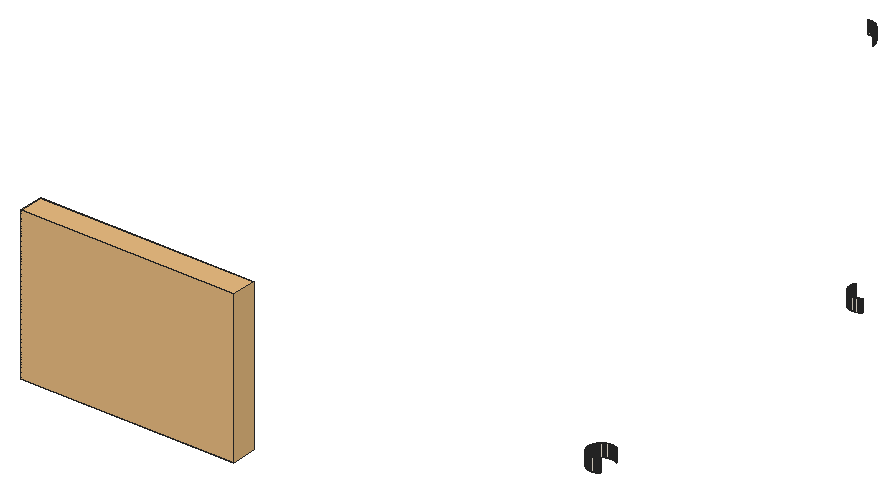
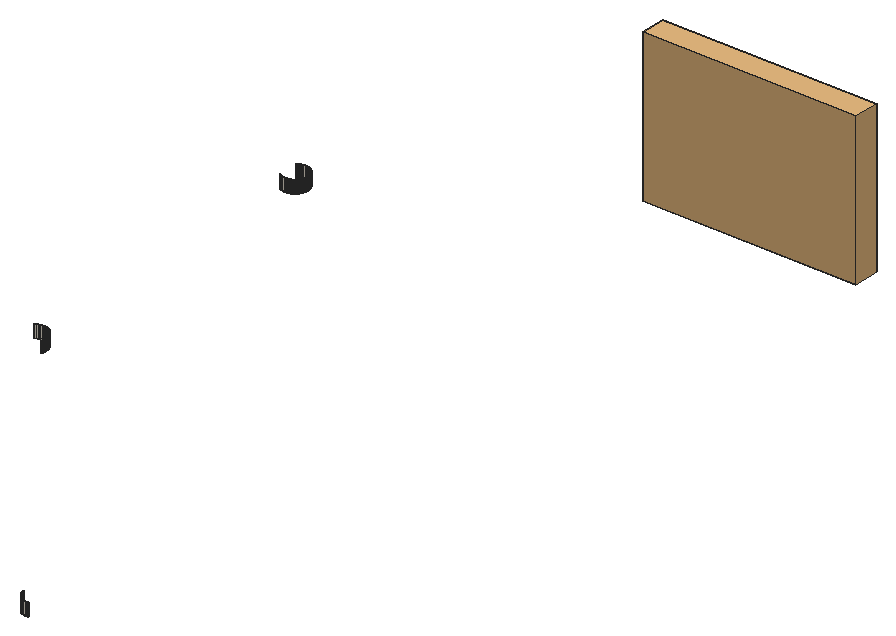
# SketchUp Ruby script. Lengths in inches.
U = 1.inch
M = Sketchup.active_model
def pt(a) = Geom::Point3d.new(a.map { |v| v * U })
def face(e, loops, mat)
  f = e.add_face(loops[0].map { |a| pt(a) })
  loops[1..].each { |l| e.add_face(l.map { |a| pt(a) }).erase! }
  f.material = f.back_material = mat if mat
  f
end
# faces: each face lists its corners as indices into pts; further lists are holes
def faces(e, pts, list, mat = nil) = list.each { |f| face(e, (f[0].is_a?(Array) ? f : [f]).map { |l| l.map { |i| pts[i] } }, mat) }
# xy, xz, yz: faces in a plane at the given z, y or x. An outline is a flat list of corners, or four numbers for a rectangle; further outlines are holes
def ring(l) = l.size == 4 ? [[l[0], l[1]], [l[2], l[1]], [l[2], l[3]], [l[0], l[3]]] : l.each_slice(2).to_a
def flat(e, list, mat, &to3) = list.each { |f| face(e, (f[0].is_a?(Array) ? f : [f]).map { |l| ring(l).map { |u, v| to3.(u, v) } }, mat) }
def xy(e, z, list, mat = nil) = flat(e, list, mat) { |x, y| [x, y, z] }
def xz(e, y, list, mat = nil) = flat(e, list, mat) { |x, z| [x, y, z] }
def yz(e, x, list, mat = nil) = flat(e, list, mat) { |y, z| [x, y, z] }
def lines(e, pts, list) = list.each { |a, b| e.add_line(pt(pts[a]), pt(pts[b])) }
# prism: a flat outline (further loops are holes) pulled along v
def prism(e, loops, v, mat = nil)
  f = face(e, loops, mat); d = Geom::Vector3d.new(v.map { |x| x * U })
  f.pushpull(f.normal.samedirection?(d) ? d.length : -d.length)
end
def box(e, o, s, mat = nil) = prism(e, [[o, [o[0] + s[0], o[1], o[2]], [o[0] + s[0], o[1] + s[1], o[2]], [o[0], o[1] + s[1], o[2]]]], [0, 0, s[2]], mat)
def at(x, y, z, deg = 0) = Geom::Transformation.translation(pt([x, y, z])) * Geom::Transformation.rotation(ORIGIN, Z_AXIS, deg.degrees)
def axes(o, x, y, z) = Geom::Transformation.new([*x, 0, *y, 0, *z, 0, *pt(o).to_a, 1])
def part(name) = M.definitions.add(name)
# library, detail: a bought-in or finely detailed component or shape, given as its bounding box
def library(name, o, s) = part(name).tap { |d| box(d.entities, o, s) }
def detail(e, o, s) = box(e.add_group.entities, o, s)
def put(e, d, t, mat = nil) = e.add_instance(d, t).tap { |i| i.material = mat if mat }
def group(e, t, mat = nil) = e.add_group.tap { |g| g.transformation = t; g.material = mat if mat }.entities
root = M.entities
M.materials.add("0027 AP L140 CRUSHED ICE").color = [241, 233, 217]
c1 = library("Group\#28",[0,0,-12],[51,6,35.99])
xz(root,255,[[122.84,120,122.92,123],[122.92,120,123,123],[123,120,123.08,123],[123.08,120,123.16,123]],"0027 AP L140 CRUSHED ICE")
xz(root,261,[[122.84,120,122.92,123],[122.92,120,123,123],[123,120,123.08,123],[123.08,120,123.16,123]],"0027 AP L140 CRUSHED ICE")
xz(root,333,[[122.84,120,122.92,123],[122.92,120,123,123],[123,120,123.08,123],[123.08,120,123.16,123]],"0027 AP L140 CRUSHED ICE")
xz(root,417,[[59.84,120,59.92,123],[59.92,120,60,123],[60,120,60.08,123],[60.08,120,60.16,123]],"0027 AP L140 CRUSHED ICE")
yz(root,63,[[414,120,414.08,123],[414.08,120,414.16,123]],"0027 AP L140 CRUSHED ICE")
yz(root,120,[[257.84,120,257.92,123],[257.92,120,258,123],[258,120,258.08,123],[258.08,120,258.16,123],[335.84,120,335.92,123],
  [335.92,120,336,123],[336,120,336.08,123],[336.08,120,336.16,123]],"0027 AP L140 CRUSHED ICE")
p = [[122.53,255.04,120],[122.45,255.05,120],[122.45,255.05,123],[122.53,255.04,123],[122.61,255.03,120],[122.61,255.03,123],
  [122.6875,255.02,120],[122.6875,255.02,123],[122.76,255.01,120],[122.76,255.01,123],[122.84,255,120],[122.84,255,123],
  [123.24,255.01,120],[123.16,255,120],[123.16,255,123],[123.24,255.01,123],[123.3125,255.02,120],[123.3125,255.02,123],
  [123.39,255.03,120],[123.39,255.03,123],[123.47,255.04,120],[123.47,255.04,123],[123.55,255.05,120],[123.55,255.05,123],
  [122.07,255.15,120],[122,255.17,120],[122,255.17,123],[122.07,255.15,123],[122.15,255.125,120],[122.15,255.125,123],
  [122.22,255.1,120],[122.22,255.1,123],[122.3,255.08,120],[122.3,255.08,123],[122.375,255.07,120],[122.375,255.07,123],
  [123.625,255.07,120],[123.625,255.07,123],[123.7,255.08,120],[123.7,255.08,123],[123.78,255.1,120],[123.78,255.1,123],
  [123.85,255.125,120],[123.85,255.125,123],[123.93,255.15,120],[123.93,255.15,123],[124,255.17,120],[124,255.17,123],
  [121.85,255.23,120],[121.78,255.26,120],[121.78,255.26,123],[121.85,255.23,123],[121.92,255.2,120],[121.92,255.2,123],
  [124.08,255.2,120],[124.08,255.2,123],[124.15,255.23,120],[124.15,255.23,123],[124.22,255.26,120],[124.22,255.26,123],
  [121.64,255.33,120],[121.57,255.36,120],[121.57,255.36,123],[121.64,255.33,123],[121.71,255.29,120],[121.71,255.29,123],
  [124.29,255.29,120],[124.29,255.29,123],[124.36,255.33,120],[124.36,255.33,123],[124.43,255.36,120],[124.43,255.36,123],
  [121.43,255.44,120],[121.37,255.48,120],[121.37,255.48,123],[121.43,255.44,123],[121.5,255.4,120],[121.5,255.4,123],
  [124.5,255.4,120],[124.5,255.4,123],[124.57,255.44,120],[124.57,255.44,123],[124.63,255.48,120],[124.63,255.48,123],
  [121.3,255.53,120],[121.24,255.57,120],[121.24,255.57,123],[121.3,255.53,123],[124.7,255.53,120],[124.7,255.53,123],
  [124.76,255.57,120],[124.76,255.57,123],[121.17,255.62,120],[121.11,255.67,120],[121.11,255.67,123],[121.17,255.62,123],
  [124.83,255.62,120],[124.83,255.62,123],[124.89,255.67,120],[124.89,255.67,123],[121.05,255.72,120],[120.99,255.77,120],
  [120.99,255.77,123],[121.05,255.72,123],[120.93,255.82,120],[120.88,255.88,120],[120.88,255.88,123],[120.93,255.82,123],
  [120.82,255.93,120],[120.77,255.99,120],[120.77,255.99,123],[120.82,255.93,123],[120.72,256.05,120],[120.72,256.05,123],
  [120.67,256.11,120],[120.62,256.17,120],[120.62,256.17,123],[120.67,256.11,123],[120.57,256.24,120],[120.53,256.3,120],
  [120.53,256.3,123],[120.57,256.24,123],[120.48,256.37,120],[120.48,256.37,123],[120.44,256.43,120],[120.4,256.5,120],
  [120.4,256.5,123],[120.44,256.43,123],[120.36,256.57,120],[120.36,256.57,123],[120.33,256.64,120],[120.29,256.71,120],
  [120.29,256.71,123],[120.33,256.64,123],[120.26,256.78,120],[120.26,256.78,123],[120.23,256.85,120],[120.23,256.85,123],
  [120.2,256.92,120],[120.17,257,120],[120.17,257,123],[120.2,256.92,123],[120.15,257.07,120],[120.15,257.07,123],
  [120.125,257.15,120],[120.1,257.22,120],[120.1,257.22,123],[120.125,257.15,123],[120.08,257.3,120],[120.08,257.3,123],
  [120.07,257.375,120],[120.07,257.375,123],[120.05,257.45,120],[120.05,257.45,123],[120.04,257.53,120],[120.03,257.61,120],
  [120.03,257.61,123],[120.04,257.53,123],[120.02,257.6875,120],[120.02,257.6875,123],[120.01,257.76,120],[120.01,257.76,123],
  [120,257.84,120],[120,257.84,123],[120,258.16,120],[120.01,258.24,120],[120.01,258.24,123],[120,258.16,123],
  [120.02,258.3125,120],[120.02,258.3125,123],[120.03,258.39,120],[120.03,258.39,123],[120.04,258.47,120],[120.04,258.47,123],
  [120.05,258.55,120],[120.05,258.55,123],[120.07,258.625,120],[120.07,258.625,123],[120.08,258.7,120],[120.08,258.7,123],
  [120.1,258.78,120],[120.1,258.78,123],[120.125,258.85,120],[120.125,258.85,123],[120.15,258.93,120],[120.15,258.93,123],
  [120.17,259,120],[120.17,259,123],[120.2,259.08,120],[120.2,259.08,123],[120.23,259.15,120],[120.23,259.15,123],
  [120.26,259.22,120],[120.26,259.22,123],[120.29,259.29,120],[120.29,259.29,123],[120.33,259.36,120],[120.33,259.36,123],
  [120.36,259.43,120],[120.36,259.43,123],[120.4,259.5,120],[120.4,259.5,123],[120.44,259.57,120],[120.44,259.57,123],
  [120.48,259.63,120],[120.48,259.63,123],[120.53,259.7,120],[120.53,259.7,123],[120.57,259.76,120],[120.57,259.76,123],
  [120.62,259.83,120],[120.62,259.83,123],[120.67,259.89,120],[120.67,259.89,123],[120.72,259.95,120],[120.72,259.95,123],
  [120.77,260.01,120],[120.77,260.01,123],[120.82,260.07,120],[120.82,260.07,123],[120.88,260.12,120],[120.88,260.12,123],
  [120.93,260.18,120],[120.93,260.18,123],[120.99,260.23,120],[120.99,260.23,123],[121.05,260.28,120],[121.05,260.28,123],
  [121.11,260.33,120],[121.11,260.33,123],[121.17,260.38,120],[121.17,260.38,123],[124.83,260.38,120],[124.89,260.33,120],
  [124.89,260.33,123],[124.83,260.38,123],[121.24,260.43,120],[121.24,260.43,123],[121.3,260.47,120],[121.3,260.47,123],
  [124.7,260.47,120],[124.76,260.43,120],[124.76,260.43,123],[124.7,260.47,123],[121.37,260.52,120],[121.37,260.52,123],
  [121.43,260.56,120],[121.43,260.56,123],[124.57,260.56,120],[124.63,260.52,120],[124.63,260.52,123],[124.57,260.56,123],
  [121.5,260.6,120],[121.5,260.6,123],[121.57,260.64,120],[121.57,260.64,123],[121.64,260.67,120],[121.64,260.67,123],
  [124.36,260.67,120],[124.43,260.64,120],[124.43,260.64,123],[124.36,260.67,123],[124.5,260.6,120],[124.5,260.6,123],
  [121.71,260.71,120],[121.71,260.71,123],[121.78,260.74,120],[121.78,260.74,123],[121.85,260.77,120],[121.85,260.77,123],
  [124.15,260.77,120],[124.22,260.74,120],[124.22,260.74,123],[124.15,260.77,123],[124.29,260.71,120],[124.29,260.71,123],
  [121.92,260.8,120],[121.92,260.8,123],[122,260.83,120],[122,260.83,123],[122.07,260.85,120],[122.07,260.85,123],
  [123.93,260.85,120],[124,260.83,120],[124,260.83,123],[123.93,260.85,123],[124.08,260.8,120],[124.08,260.8,123],
  [122.15,260.875,120],[122.15,260.875,123],[122.22,260.9,120],[122.22,260.9,123],[122.3,260.92,120],[122.3,260.92,123],
  [122.375,260.93,120],[122.375,260.93,123],[122.45,260.95,120],[122.45,260.95,123],[122.53,260.96,120],[122.53,260.96,123],
  [123.47,260.96,120],[123.55,260.95,120],[123.55,260.95,123],[123.47,260.96,123],[123.625,260.93,120],[123.625,260.93,123],
  [123.7,260.92,120],[123.7,260.92,123],[123.78,260.9,120],[123.78,260.9,123],[123.85,260.875,120],[123.85,260.875,123],
  [122.61,260.97,120],[122.61,260.97,123],[122.6875,260.98,120],[122.6875,260.98,123],[122.76,260.99,120],[122.76,260.99,123],
  [122.84,261,120],[122.84,261,123],[123.16,261,120],[123.24,260.99,120],[123.24,260.99,123],[123.16,261,123],
  [123.3125,260.98,120],[123.3125,260.98,123],[123.39,260.97,120],[123.39,260.97,123],[122.53,333.04,120],[122.45,333.05,120],
  [122.45,333.05,123],[122.53,333.04,123],[122.61,333.03,120],[122.61,333.03,123],[122.6875,333.02,120],[122.6875,333.02,123],
  [122.76,333.01,120],[122.76,333.01,123],[122.84,333,120],[122.84,333,123],[123.24,333.01,120],[123.16,333,120],
  [123.16,333,123],[123.24,333.01,123],[123.3125,333.02,120],[123.3125,333.02,123],[123.39,333.03,120],[123.39,333.03,123],
  [123.47,333.04,120],[123.47,333.04,123],[123.55,333.05,120],[123.55,333.05,123],[122.07,333.15,120],[122,333.17,120],
  [122,333.17,123],[122.07,333.15,123],[122.15,333.125,120],[122.15,333.125,123],[122.22,333.1,120],[122.22,333.1,123],
  [122.3,333.08,120],[122.3,333.08,123],[122.375,333.07,120],[122.375,333.07,123],[123.625,333.07,120],[123.625,333.07,123],
  [123.7,333.08,120],[123.7,333.08,123],[123.78,333.1,120],[123.78,333.1,123],[123.85,333.125,120],[123.85,333.125,123],
  [123.93,333.15,120],[123.93,333.15,123],[124,333.17,120],[124,333.17,123],[121.85,333.23,120],[121.78,333.26,120],
  [121.78,333.26,123],[121.85,333.23,123],[121.92,333.2,120],[121.92,333.2,123],[124.08,333.2,120],[124.08,333.2,123],
  [124.15,333.23,120],[124.15,333.23,123],[124.22,333.26,120],[124.22,333.26,123],[121.64,333.33,120],[121.57,333.36,120],
  [121.57,333.36,123],[121.64,333.33,123],[121.71,333.29,120],[121.71,333.29,123],[124.29,333.29,120],[124.29,333.29,123],
  [124.36,333.33,120],[124.36,333.33,123],[124.43,333.36,120],[124.43,333.36,123],[121.43,333.44,120],[121.37,333.48,120],
  [121.37,333.48,123],[121.43,333.44,123],[121.5,333.4,120],[121.5,333.4,123],[124.5,333.4,120],[124.5,333.4,123],
  [124.57,333.44,120],[124.57,333.44,123],[124.63,333.48,120],[124.63,333.48,123],[121.3,333.53,120],[121.24,333.57,120],
  [121.24,333.57,123],[121.3,333.53,123],[124.7,333.53,120],[124.7,333.53,123],[124.76,333.57,120],[124.76,333.57,123],
  [121.17,333.62,120],[121.11,333.67,120],[121.11,333.67,123],[121.17,333.62,123],[124.83,333.62,120],[124.83,333.62,123],
  [124.89,333.67,120],[124.89,333.67,123],[121.05,333.72,120],[120.99,333.77,120],[120.99,333.77,123],[121.05,333.72,123],
  [120.93,333.82,120],[120.88,333.88,120],[120.88,333.88,123],[120.93,333.82,123],[120.82,333.93,120],[120.77,333.99,120],
  [120.77,333.99,123],[120.82,333.93,123],[120.72,334.05,120],[120.72,334.05,123],[120.67,334.11,120],[120.62,334.17,120],
  [120.62,334.17,123],[120.67,334.11,123],[120.57,334.24,120],[120.53,334.3,120],[120.53,334.3,123],[120.57,334.24,123],
  [120.48,334.37,120],[120.48,334.37,123],[120.44,334.43,120],[120.4,334.5,120],[120.4,334.5,123],[120.44,334.43,123],
  [120.36,334.57,120],[120.36,334.57,123],[120.33,334.64,120],[120.29,334.71,120],[120.29,334.71,123],[120.33,334.64,123],
  [120.26,334.78,120],[120.26,334.78,123],[120.23,334.85,120],[120.23,334.85,123],[120.2,334.92,120],[120.17,335,120],
  [120.17,335,123],[120.2,334.92,123],[120.15,335.07,120],[120.15,335.07,123],[120.125,335.15,120],[120.1,335.22,120],
  [120.1,335.22,123],[120.125,335.15,123],[120.08,335.3,120],[120.08,335.3,123],[120.07,335.375,120],[120.07,335.375,123],
  [120.05,335.45,120],[120.05,335.45,123],[120.04,335.53,120],[120.03,335.61,120],[120.03,335.61,123],[120.04,335.53,123],
  [120.02,335.6875,120],[120.02,335.6875,123],[120.01,335.76,120],[120.01,335.76,123],[120,335.84,120],[120,335.84,123],
  [120,336.16,120],[120.01,336.24,120],[120.01,336.24,123],[120,336.16,123],[120.02,336.3125,120],[120.02,336.3125,123],
  [120.03,336.39,120],[120.03,336.39,123],[120.04,336.47,120],[120.04,336.47,123],[120.05,336.55,120],[120.05,336.55,123],
  [120.07,336.625,120],[120.07,336.625,123],[120.08,336.7,120],[120.08,336.7,123],[120.1,336.78,120],[120.1,336.78,123],
  [120.125,336.85,120],[120.125,336.85,123],[120.15,336.93,120],[120.15,336.93,123],[120.17,337,120],[120.17,337,123],
  [120.2,337.08,120],[120.2,337.08,123],[120.23,337.15,120],[120.23,337.15,123],[120.26,337.22,120],[120.26,337.22,123],
  [62.98,414.3125,120],[62.99,414.24,120],[62.99,414.24,123],[62.98,414.3125,123],[63,414.16,120],[63,414.16,123],
  [62.97,414.39,120],[62.97,414.39,123],[62.96,414.47,120],[62.96,414.47,123],[62.93,414.625,120],[62.95,414.55,120],
  [62.95,414.55,123],[62.93,414.625,123],[62.92,414.7,120],[62.92,414.7,123],[62.9,414.78,120],[62.9,414.78,123],
  [62.875,414.85,120],[62.875,414.85,123],[62.83,415,120],[62.85,414.93,120],[62.85,414.93,123],[62.83,415,123],
  [62.8,415.08,120],[62.8,415.08,123],[62.74,415.22,120],[62.77,415.15,120],[62.77,415.15,123],[62.74,415.22,123],
  [62.71,415.29,120],[62.71,415.29,123],[62.67,415.36,120],[62.67,415.36,123],[62.6,415.5,120],[62.64,415.43,120],
  [62.64,415.43,123],[62.6,415.5,123],[62.56,415.57,120],[62.56,415.57,123],[62.47,415.7,120],[62.52,415.63,120],
  [62.52,415.63,123],[62.47,415.7,123],[62.43,415.76,120],[62.43,415.76,123],[62.33,415.89,120],[62.38,415.83,120],
  [62.38,415.83,123],[62.33,415.89,123],[62.23,416.01,120],[62.28,415.95,120],[62.28,415.95,123],[62.23,416.01,123],
  [62.18,416.07,120],[62.18,416.07,123],[62.07,416.18,120],[62.12,416.12,120],[62.12,416.12,123],[62.07,416.18,123],
  [61.95,416.28,120],[62.01,416.23,120],[62.01,416.23,123],[61.95,416.28,123],[61.83,416.38,120],[61.89,416.33,120],
  [61.89,416.33,123],[61.83,416.38,123],[61.7,416.47,120],[61.76,416.43,120],[61.76,416.43,123],[61.7,416.47,123],
  [61.57,416.56,120],[61.63,416.52,120],[61.63,416.52,123],[61.57,416.56,123],[61.36,416.67,120],[61.43,416.64,120],
  [61.43,416.64,123],[61.36,416.67,123],[61.5,416.6,120],[61.5,416.6,123],[61.15,416.77,120],[61.22,416.74,120],
  [61.22,416.74,123],[61.15,416.77,123],[61.29,416.71,120],[61.29,416.71,123],[60.93,416.85,120],[61,416.83,120],
  [61,416.83,123],[60.93,416.85,123],[61.08,416.8,120],[61.08,416.8,123],[59.375,416.93,120],[59.45,416.95,120],
  [59.45,416.95,123],[59.375,416.93,123],[59.53,416.96,120],[59.53,416.96,123],[60.47,416.96,120],[60.55,416.95,120],
  [60.55,416.95,123],[60.47,416.96,123],[60.625,416.93,120],[60.625,416.93,123],[60.7,416.92,120],[60.7,416.92,123],
  [60.78,416.9,120],[60.78,416.9,123],[60.85,416.875,120],[60.85,416.875,123],[59.61,416.97,120],[59.61,416.97,123],
  [59.6875,416.98,120],[59.6875,416.98,123],[59.76,416.99,120],[59.76,416.99,123],[59.84,417,120],[59.84,417,123],
  [60.16,417,120],[60.24,416.99,120],[60.24,416.99,123],[60.16,417,123],[60.3125,416.98,120],[60.3125,416.98,123],
  [60.39,416.97,120],[60.39,416.97,123]]
faces(root,p,[[0,1,2,3],[4,0,3,5],[6,4,5,7],[8,6,7,9],[10,8,9,11],[12,13,14,15],[16,12,15,17],[18,16,17,19],
  [20,18,19,21],[22,20,21,23],[24,25,26,27],[28,24,27,29],[30,28,29,31],[32,30,31,33],[34,32,33,35],[1,34,35,2],
  [36,22,23,37],[38,36,37,39],[40,38,39,41],[42,40,41,43],[44,42,43,45],[46,44,45,47],[48,49,50,51],[52,48,51,53],
  [25,52,53,26],[54,46,47,55],[56,54,55,57],[58,56,57,59],[60,61,62,63],[64,60,63,65],[49,64,65,50],[66,58,59,67],
  [68,66,67,69],[70,68,69,71],[72,73,74,75],[76,72,75,77],[61,76,77,62],[78,70,71,79],[80,78,79,81],[82,80,81,83],
  [84,85,86,87],[73,84,87,74],[88,82,83,89],[90,88,89,91],[92,93,94,95],[85,92,95,86],[96,90,91,97],[98,96,97,99],
  [100,101,102,103],[93,100,103,94],[104,105,106,107],[101,104,107,102],[108,109,110,111],[105,108,111,106],[109,112,113,110],[114,115,116,117],
  [112,114,117,113],[118,119,120,121],[115,118,121,116],[119,122,123,120],[124,125,126,127],[122,124,127,123],[125,128,129,126],[130,131,132,133],
  [128,130,133,129],[131,134,135,132],[134,136,137,135],[138,139,140,141],[136,138,141,137],[139,142,143,140],[144,145,146,147],[142,144,147,143],
  [145,148,149,146],[148,150,151,149],[150,152,153,151],[154,155,156,157],[152,154,157,153],[155,158,159,156],[158,160,161,159],[160,162,163,161],
  [164,165,166,167],[165,168,169,166],[168,170,171,169],[170,172,173,171],[172,174,175,173],[174,176,177,175],[176,178,179,177],[178,180,181,179],
  [180,182,183,181],[182,184,185,183],[184,186,187,185],[186,188,189,187],[188,190,191,189],[190,192,193,191],[192,194,195,193],[194,196,197,195],
  [196,198,199,197],[198,200,201,199],[200,202,203,201],[202,204,205,203],[204,206,207,205],[206,208,209,207],[208,210,211,209],[210,212,213,211],
  [212,214,215,213],[214,216,217,215],[216,218,219,217],[218,220,221,219],[220,222,223,221],[222,224,225,223],[224,226,227,225],[226,228,229,227],
  [228,230,231,229],[232,233,234,235],[230,236,237,231],[236,238,239,237],[240,241,242,243],[241,232,235,242],[238,244,245,239],[244,246,247,245],
  [248,249,250,251],[249,240,243,250],[246,252,253,247],[252,254,255,253],[254,256,257,255],[258,259,260,261],[259,262,263,260],[262,248,251,263],
  [256,264,265,257],[264,266,267,265],[266,268,269,267],[270,271,272,273],[271,274,275,272],[274,258,261,275],[268,276,277,269],[276,278,279,277],
  [278,280,281,279],[282,283,284,285],[283,286,287,284],[286,270,273,287],[280,288,289,281],[288,290,291,289],[290,292,293,291],[292,294,295,293],
  [294,296,297,295],[296,298,299,297],[300,301,302,303],[301,304,305,302],[304,306,307,305],[306,308,309,307],[308,310,311,309],[310,282,285,311],
  [298,312,313,299],[312,314,315,313],[314,316,317,315],[316,318,319,317],[320,321,322,323],[321,324,325,322],[324,326,327,325],[326,300,303,327],
  [328,329,330,331],[332,328,331,333],[334,332,333,335],[336,334,335,337],[338,336,337,339],[340,341,342,343],[344,340,343,345],[346,344,345,347],
  [348,346,347,349],[350,348,349,351],[352,353,354,355],[356,352,355,357],[358,356,357,359],[360,358,359,361],[362,360,361,363],[329,362,363,330],
  [364,350,351,365],[366,364,365,367],[368,366,367,369],[370,368,369,371],[372,370,371,373],[374,372,373,375],[376,377,378,379],[380,376,379,381],
  [353,380,381,354],[382,374,375,383],[384,382,383,385],[386,384,385,387],[388,389,390,391],[392,388,391,393],[377,392,393,378],[394,386,387,395],
  [396,394,395,397],[398,396,397,399],[400,401,402,403],[404,400,403,405],[389,404,405,390],[406,398,399,407],[408,406,407,409],[410,408,409,411],
  [412,413,414,415],[401,412,415,402],[416,410,411,417],[418,416,417,419],[420,421,422,423],[413,420,423,414],[424,418,419,425],[426,424,425,427],
  [428,429,430,431],[421,428,431,422],[432,433,434,435],[429,432,435,430],[436,437,438,439],[433,436,439,434],[437,440,441,438],[442,443,444,445],
  [440,442,445,441],[446,447,448,449],[443,446,449,444],[447,450,451,448],[452,453,454,455],[450,452,455,451],[453,456,457,454],[458,459,460,461],
  [456,458,461,457],[459,462,463,460],[462,464,465,463],[466,467,468,469],[464,466,469,465],[467,470,471,468],[472,473,474,475],[470,472,475,471],
  [473,476,477,474],[476,478,479,477],[478,480,481,479],[482,483,484,485],[480,482,485,481],[483,486,487,484],[486,488,489,487],[488,490,491,489],
  [492,493,494,495],[493,496,497,494],[496,498,499,497],[498,500,501,499],[500,502,503,501],[502,504,505,503],[504,506,507,505],[506,508,509,507],
  [508,510,511,509],[510,512,513,511],[512,514,515,513],[514,516,517,515],[516,518,519,517],[518,520,521,519],[522,523,524,525],[523,526,527,524],
  [528,522,525,529],[530,528,529,531],[532,533,534,535],[533,530,531,534],[536,532,535,537],[538,536,537,539],[540,538,539,541],[542,543,544,545],
  [543,540,541,544],[546,542,545,547],[548,549,550,551],[549,546,547,550],[552,548,551,553],[554,552,553,555],[556,557,558,559],[557,554,555,558],
  [560,556,559,561],[562,563,564,565],[563,560,561,564],[566,562,565,567],[568,569,570,571],[569,566,567,570],[572,573,574,575],[573,568,571,574],
  [576,572,575,577],[578,579,580,581],[579,576,577,580],[582,583,584,585],[583,578,581,584],[586,587,588,589],[587,582,585,588],[590,591,592,593],
  [591,586,589,592],[594,595,596,597],[595,590,593,596],[598,599,600,601],[599,602,603,600],[602,594,597,603],[604,605,606,607],[605,608,609,606],
  [608,598,601,609],[610,611,612,613],[611,614,615,612],[614,604,607,615],[616,617,618,619],[617,620,621,618],[622,623,624,625],[623,626,627,624],
  [626,628,629,627],[628,630,631,629],[630,632,633,631],[632,610,613,633],[620,634,635,621],[634,636,637,635],[636,638,639,637],[638,640,641,639],
  [642,643,644,645],[643,646,647,644],[646,648,649,647],[648,622,625,649]],"0027 AP L140 CRUSHED ICE")
put(root,c1,at(18,216,132),"0027 AP L140 CRUSHED ICE")
